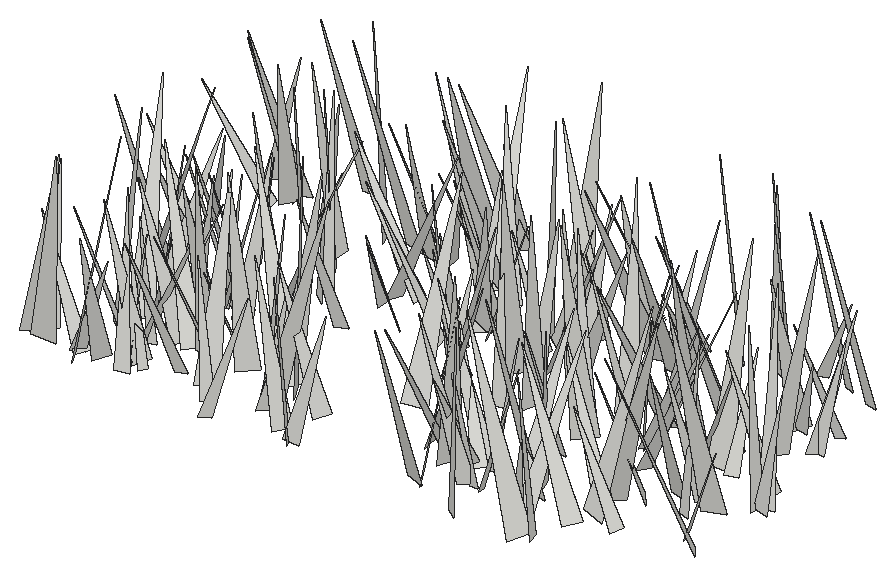
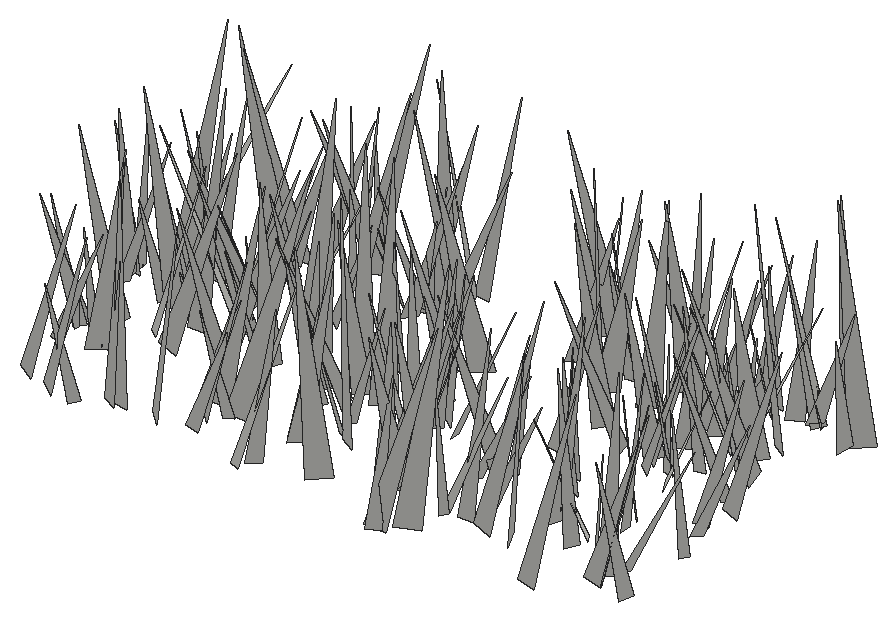
# SketchUp Ruby script. Lengths in inches.
U = 1.inch
M = Sketchup.active_model
def pt(a) = Geom::Point3d.new(a.map { |v| v * U })
def face(e, loops, mat)
  f = e.add_face(loops[0].map { |a| pt(a) })
  loops[1..].each { |l| e.add_face(l.map { |a| pt(a) }).erase! }
  f.material = f.back_material = mat if mat
  f
end
# faces: each face lists its corners as indices into pts; further lists are holes
def faces(e, pts, list, mat = nil) = list.each { |f| face(e, (f[0].is_a?(Array) ? f : [f]).map { |l| l.map { |i| pts[i] } }, mat) }
# xy, xz, yz: faces in a plane at the given z, y or x. An outline is a flat list of corners, or four numbers for a rectangle; further outlines are holes
def ring(l) = l.size == 4 ? [[l[0], l[1]], [l[2], l[1]], [l[2], l[3]], [l[0], l[3]]] : l.each_slice(2).to_a
def flat(e, list, mat, &to3) = list.each { |f| face(e, (f[0].is_a?(Array) ? f : [f]).map { |l| ring(l).map { |u, v| to3.(u, v) } }, mat) }
def xy(e, z, list, mat = nil) = flat(e, list, mat) { |x, y| [x, y, z] }
def xz(e, y, list, mat = nil) = flat(e, list, mat) { |x, z| [x, y, z] }
def yz(e, x, list, mat = nil) = flat(e, list, mat) { |y, z| [x, y, z] }
def lines(e, pts, list) = list.each { |a, b| e.add_line(pt(pts[a]), pt(pts[b])) }
# prism: a flat outline (further loops are holes) pulled along v
def prism(e, loops, v, mat = nil)
  f = face(e, loops, mat); d = Geom::Vector3d.new(v.map { |x| x * U })
  f.pushpull(f.normal.samedirection?(d) ? d.length : -d.length)
end
def box(e, o, s, mat = nil) = prism(e, [[o, [o[0] + s[0], o[1], o[2]], [o[0] + s[0], o[1] + s[1], o[2]], [o[0], o[1] + s[1], o[2]]]], [0, 0, s[2]], mat)
def at(x, y, z, deg = 0) = Geom::Transformation.translation(pt([x, y, z])) * Geom::Transformation.rotation(ORIGIN, Z_AXIS, deg.degrees)
def axes(o, x, y, z) = Geom::Transformation.new([*x, 0, *y, 0, *z, 0, *pt(o).to_a, 1])
def part(name) = M.definitions.add(name)
# library, detail: a bought-in or finely detailed component or shape, given as its bounding box
def library(name, o, s) = part(name).tap { |d| box(d.entities, o, s) }
def detail(e, o, s) = box(e.add_group.entities, o, s)
def put(e, d, t, mat = nil) = e.add_instance(d, t).tap { |i| i.material = mat if mat }
def group(e, t, mat = nil) = e.add_group.tap { |g| g.transformation = t; g.material = mat if mat }.entities
root = M.entities
c1 = part("fur_instance\#9")
p = [[0.8125,0,1.79],[0.67,-0.02,1.48],[0,-0.11,0],[0,0.11,0]]
faces(c1.entities,p,[[0,1,2,3]])
put(root,c1,axes([529.7,255.59,-21.66],[-1.86711,-6.21996,0.83765],[-6.21183,1.95621,0.67975],[0.89595,0.60083,6.45848]))
put(root,c1,axes([505.19,255.6,-21.66],[4.3108,-3.69492,0.61953],[-3.55093,-4.33068,-1.12044],[-1.19463,-0.46051,5.56597]))
put(root,c1,axes([539.13,253.99,-21.66],[-7.00283,2.97011,1.6591],[3.21934,7.01289,1.03394],[1.10002,-1.61605,7.53606]))
put(root,c1,axes([500.92,255.19,-21.66],[1.84601,-7.44066,1.73932],[-7.59322,-1.58595,1.27441],[0.85535,1.97933,7.55956]))
put(root,c1,axes([499.92,255.59,-21.66],[4.60789,-6.31495,1.14074],[-6.41656,-4.51508,0.92427],[0.08686,1.46561,7.76253]))
put(root,c1,axes([534.02,253.74,-21.66],[3.38997,4.6985,2.258],[4.82742,-3.84601,0.75539],[-1.96736,-1.34115,5.74432]))
put(root,c1,axes([514.75,253.74,-21.66],[3.82826,-1.89723,1.31218],[-2.241,-3.66166,1.2438],[-0.54703,1.72325,4.08754]))
put(root,c1,axes([503.53,255.34,-21.66],[3.31192,-3.28223,0.0309],[-3.2384,-3.26025,0.79144],[0.53549,0.5836,4.59516]))
put(root,c1,axes([520.81,254.58,-21.66],[1.98838,-4.24744,1.75797],[-4.57109,-1.62434,1.24561],[0.4862,2.09896,4.52138]))
put(root,c1,axes([520.7,254.41,-21.66],[-4.62696,-2.40171,1.71965],[-2.7299,4.69747,-0.78458],[1.12828,1.51649,5.15378]))
put(root,c1,axes([539.83,254.45,-21.66],[-4.89428,-1.48699,1.50253],[-1.73277,4.99254,-0.70337],[1.21087,1.13406,5.0666]))
put(root,c1,axes([537.2,256.21,-21.66],[0.94706,-3.59902,0.23008],[-3.53322,-0.8783,0.80484],[0.72266,0.42244,3.63347]))
put(root,c1,axes([519.43,255.46,-21.66],[-4.54367,3.48057,1.82928],[3.81076,4.58683,0.73803],[0.96889,-1.71821,5.67579]))
put(root,c1,axes([503.85,255.37,-21.66],[-3.48001,3.233,0.8636],[3.33945,3.27515,1.19585],[-0.21495,-1.45934,4.59703]))
put(root,c1,axes([529.92,255.99,-21.66],[6.22111,3.48137,1.76986],[3.77865,-6.20685,-1.07301],[-0.98698,-1.81924,7.04775]))
put(root,c1,axes([510.18,257.15,-21.66],[-0.32554,-5.06602,0.7464],[-4.99056,0.14633,-1.18345],[-1.14716,0.80105,4.9366]))
put(root,c1,axes([513.71,255.28,-21.66],[-0.78367,4.54033,1.31363],[4.69244,0.5877,0.76808],[-0.56674,-1.41222,4.54299]))
put(root,c1,axes([503.8,254.6,-21.66],[6.26441,4.08516,1.86388],[4.05019,-6.52197,0.68206],[-1.9387,-0.42509,7.44756]))
put(root,c1,axes([507.48,256.67,-21.66],[-4.95355,2.49117,1.9463],[2.93301,4.97148,1.10159],[1.17959,-1.90003,5.43416]))
put(root,c1,axes([507.28,254.95,-21.66],[-0.20928,5.81187,1.2771],[5.90875,0.05179,0.73257],[-0.70395,-1.2931,5.76932]))
put(root,c1,axes([532.45,257.21,-21.66],[0.82361,-5.861,1.93807],[-5.93962,-1.28507,-1.3621],[-1.68178,1.66825,5.75972]))
put(root,c1,axes([506.9,256.625,-21.66],[-4.69197,-2.31538,0.05263],[-2.28134,4.60011,-1.00642],[-0.39908,0.92541,5.13447]))
put(root,c1,axes([508.08,255.99,-21.66],[-3.93894,0.78438,0.2139],[0.7314,3.88076,-0.76228],[0.35506,0.70765,3.94328]))
put(root,c1,axes([531.32,259.23,-21.66],[3.03189,-3.59681,0.02756],[-3.43565,-2.90654,-1.37057],[-1.06494,-0.8632,4.50011]))
put(root,c1,axes([510.91,259.46,-21.66],[-3.83453,-4.44323,0.31037],[-4.29048,3.7947,1.3169],[1.19597,-0.63261,5.71941]))
put(root,c1,axes([506.93,255.87,-21.66],[2.12896,3.50938,0.78952],[3.35263,-2.26833,1.04217],[-1.30344,-0.10245,3.97015]))
put(root,c1,axes([533.06,257.12,-21.66],[0.75971,3.71481,1.88794],[3.89435,-1.31575,1.02184],[-1.48263,-1.55251,3.65142]))
put(root,c1,axes([517.31,256.875,-21.66],[7.2049,-3.47591,1.96261],[-3.83046,-7.15988,1.38131],[-1.1231,2.12096,7.87937]))
put(root,c1,axes([529.9,258.76,-21.66],[6.97183,-3.45055,1.53762],[-3.37643,-7.13932,-0.71191],[-1.69419,0.0288,7.74635]))
put(root,c1,axes([529.5,259.22,-21.66],[-1.20375,-5.21342,0.24756],[-5.17288,1.15789,-0.76855],[-0.69453,0.4118,5.2951]))
put(root,c1,axes([540.64,257.33,-21.66],[-4.45803,3.98436,0.74293],[4.03358,4.25341,1.39275],[-0.39655,-1.52789,5.81458]))
put(root,c1,axes([520.36,258.25,-21.66],[-4.35819,2.96505,1.59627],[3.3258,4.19926,1.28011],[0.52792,-1.97688,5.11338]))
put(root,c1,axes([512.49,256.76,-21.66],[-3.77046,5.93467,2.17976],[6.06315,4.1134,-0.71146],[1.79161,-1.43096,6.99504]))
put(root,c1,axes([536.93,258.7,-21.66],[-2.90211,-6.23156,1.67253],[-6.44447,2.71044,-1.08359],[-0.31368,1.96803,6.78825]))
put(root,c1,axes([543.29,258.36,-21.66],[-3.79672,1.89832,0.59417],[1.98792,3.66583,0.99077],[0.06937,-1.15319,4.1276]))
put(root,c1,axes([537.78,255.93,-21.66],[0.187,6.43803,0.46404],[6.40843,-0.12967,-0.78342],[0.77175,-0.48321,6.39292]))
put(root,c1,axes([516.23,257.9,-21.66],[0.00091,-3.67707,1.93886],[-4.08733,0.35251,0.67045],[0.75747,1.90654,3.61543]))
put(root,c1,axes([500.5,256.58,-21.66],[-4.9436,1.78617,0.77223],[1.56135,4.89918,-1.33648],[1.16143,1.01666,5.08364]))
put(root,c1,axes([548.65,259.28,-21.66],[-5.4011,-4.4458,0.12135],[-4.40164,5.31613,-1.14717],[-0.63674,0.96192,6.9008]))
put(root,c1,axes([533.65,257.16,-21.66],[3.84083,1.33111,0.88578],[1.09907,-3.87194,1.0529],[-1.16125,0.73803,3.92622]))
put(root,c1,axes([510.02,259.74,-21.66],[-0.4517,-7.27096,2.0225],[-7.50286,0.65147,0.6664],[0.81515,1.96726,7.25444]))
put(root,c1,axes([516.55,257.27,-21.66],[3.29752,4.92899,1.52703],[4.76096,-3.60504,1.35547],[-1.98997,-0.45731,5.77332]))
put(root,c1,axes([503.68,259.08,-21.66],[4.80804,6.17674,2.98381],[6.78482,-4.81897,-0.95722],[-1.01068,-2.96612,7.76873]))
put(root,c1,axes([536.38,259.86,-21.66],[5.52429,1.58059,2.16664],[1.98524,-5.74559,-0.8703],[-1.80317,-1.48335,5.67966]))
put(root,c1,axes([527.5,260.02,-21.66],[7.30646,0.41261,0.41525],[0.46932,-7.23653,-1.06747],[-0.34987,-1.09065,7.23983]))
put(root,c1,axes([536.5,257.24,-21.66],[-1.23708,6.4323,0.84499],[6.38548,1.35924,-0.99849],[1.14637,-0.62994,6.47363]))
put(root,c1,axes([513.18,259.92,-21.66],[3.99451,-5.40043,2.70776],[-5.64329,-4.49426,-0.63847],[-2.15638,1.75774,6.68679]))
put(root,c1,axes([506.53,258.8125,-21.66],[0.17252,3.92598,1.26935],[3.97591,-0.49782,0.99933],[-1.10305,-1.18034,3.80058]))
put(root,c1,axes([507.77,260.11,-21.66],[-5.02237,2.51021,1.68016],[2.86774,4.98644,1.12241],[0.94877,-1.78398,5.50142]))
put(root,c1,axes([539.04,259.47,-21.66],[-4.27231,-1.94809,0.06255],[-1.87913,4.07681,-1.37844],[-0.51754,1.27912,4.48861]))
put(root,c1,axes([505.97,258.65,-21.66],[4.9565,-0.0282,0.53243],[-0.1703,-4.80111,1.33099],[-0.50525,1.34155,4.77453]))
put(root,c1,axes([547,260.55,-21.66],[4.10425,1.09153,0.3293],[1.14011,-3.92312,-1.20584],[0.00571,-1.24998,4.07214]))
put(root,c1,axes([541.01,258.87,-21.66],[1.96643,7.28816,1.86053],[7.47956,-1.69089,-1.28167],[0.79683,-2.11408,7.43918]))
put(root,c1,axes([511.16,261.6,-21.66],[-2.38013,-2.88459,0.25848],[-2.75196,2.35686,0.96161],[0.90246,-0.42079,3.61403]))
put(root,c1,axes([517.23,259.52,-21.66],[6.18055,4.14964,3.19418],[4.26505,-6.85588,0.65402],[-3.03836,-1.18276,7.41558]))
put(root,c1,axes([541.47,259.5625,-21.66],[-3.45745,4.3845,0.64107],[4.38114,3.2607,1.32749],[-0.66366,-1.31634,5.42361]))
put(root,c1,axes([540.75,261.18,-21.66],[6.79044,-4.4332,0.71146],[-4.48312,-6.76549,0.63187],[-0.24718,0.91888,8.0848]))
put(root,c1,axes([531.81,259.29,-21.66],[-2.66965,3.73747,0.14274],[3.69986,2.61324,0.77338],[-0.54785,-0.56423,4.52743]))
put(root,c1,axes([531.67,260.2,-21.66],[-5.56985,2.38046,0.65327],[2.45077,5.52546,0.76123],[0.29505,-0.95874,6.00918]))
put(root,c1,axes([508.24,262.47,-21.66],[4.15376,-5.21591,0.7578],[-5.12927,-4.22232,-0.94677],[-1.21268,-0.00681,6.60024]))
put(root,c1,axes([542.1875,262.52,-21.66],[-3.97091,-3.72473,0.66515],[-3.58252,4.01146,1.07602],[1.21718,-0.34456,5.33703]))
put(root,c1,axes([508.82,259.92,-21.66],[-4.49285,4.90641,0.97236],[5.00159,4.41981,0.80831],[0.04935,-1.26349,6.60342]))
put(root,c1,axes([516.4375,260.02,-21.66],[-5.45873,5.352,1.02249],[5.44819,5.38274,0.9113],[0.08123,-1.36725,7.5902]))
put(root,c1,axes([532.74,259.44,-21.66],[1.96135,3.70682,0.36248],[3.45553,-1.96392,1.38604],[-1.38968,0.34826,3.95807]))
put(root,c1,axes([503.99,262.3125,-21.66],[3.91302,0.34843,0.25725],[0.41449,-3.69091,-1.30566],[-0.12562,-1.32482,3.70519]))
put(root,c1,axes([505.79,261.09,-21.66],[4.04604,3.23344,0.3968],[3.2461,-3.94826,-0.92578],[0.27467,-0.96906,5.09593]))
put(root,c1,axes([546.5,263.85,-21.66],[1.61042,-7.88282,1.5376],[-7.97737,-1.75156,-0.62458],[-0.92985,1.37466,8.02136]))
put(root,c1,axes([543.62,264.0625,-21.66],[-0.77388,-5.77446,0.46112],[-5.72229,0.83441,0.84559],[0.90132,0.33953,5.76439]))
put(root,c1,axes([503.95,260.98,-21.66],[-5.29033,5.65073,1.03717],[5.57546,5.38985,-0.92613],[1.38587,-0.11308,7.68509]))
put(root,c1,axes([513.87,263.45,-21.66],[5.12868,-4.19399,1.94705],[-4.5125,-5.17419,0.74098],[-1.00889,1.82269,6.58361]))
put(root,c1,axes([545.2,264.38,-21.66],[0.47741,-4.86513,1.33169],[-4.92648,-0.73691,-0.92606],[-1.08291,1.20759,4.79999]))
put(root,c1,axes([534.81,263.68,-21.66],[0.7235,3.49331,2.20248],[3.65755,-1.58024,1.30491],[-1.91742,-1.69623,3.32022]))
put(root,c1,axes([505.73,264.24,-21.66],[-0.80392,-5.00028,1.94874],[-5.12712,1.2977,1.21465],[1.58527,1.66129,4.91668]))
put(root,c1,axes([503.87,262.83,-21.66],[4.42151,2.80893,1.55928],[2.73673,-4.68252,0.67492],[-1.68278,-0.23477,5.19464]))
put(root,c1,axes([545.27,262.42,-21.66],[2.35955,4.93164,1.36493],[4.86886,-2.62618,1.07189],[-1.57426,-0.73054,5.36093]))
put(root,c1,axes([502.5,262.875,-21.66],[7.43833,2.19546,1.23858],[2.06036,-7.51855,0.95355],[-1.45225,0.57818,7.69672]))
put(root,c1,axes([509.09,264.95,-21.66],[-2.70694,-4.99144,1.16007],[-5.08628,2.45713,-1.29614],[-0.62448,1.62351,5.52829]))
put(root,c1,axes([507.4,264.74,-21.66],[5.27684,1.71083,0.85913],[1.8324,-5.24307,-0.81398],[-0.55438,-1.04563,5.4872]))
put(root,c1,axes([523.9,262.75,-21.66],[-2.77927,7.20298,1.80131],[7.21654,3.07297,-1.15349],[1.74623,-1.2353,7.63392]))
put(root,c1,axes([507.19,265.65,-21.66],[-1.65671,-3.63214,1.3485],[-3.6613,1.94738,0.7471],[1.26719,0.87797,3.92161]))
put(root,c1,axes([534.58,266.15,-21.66],[4.88048,-6.02987,2.56967],[-6.14977,-5.32095,-0.80587],[-2.26779,1.4525,7.7155]))
put(root,c1,axes([508.95,264.625,-21.66],[3.9195,-3.82723,2.46639],[-4.43668,-3.94163,0.93419],[-1.02305,2.43088,5.39791]))
put(root,c1,axes([548.6875,265.67,-21.66],[0.22976,-4.49295,1.68417],[-4.67204,0.17468,1.10336],[1.09322,1.69077,4.36142]))
put(root,c1,axes([524.9375,264.5,-21.66],[6.05583,0.88682,1.38397],[0.67013,-6.15634,1.01257],[-1.50092,0.82941,6.03608]))
put(root,c1,axes([508.51,266.19,-21.66],[-2.89225,-3.68575,0.79235],[-3.76683,2.78458,-0.79678],[-0.15371,1.11313,4.61682]))
put(root,c1,axes([511.09,265.11,-21.66],[6.06997,0.80019,0.53139],[0.73411,-6.05703,0.73529],[-0.61948,0.66277,6.07817]))
put(root,c1,axes([539.79,265.375,-21.66],[5.54197,-0.978,0.47716],[-1.05474,-5.437,1.10644],[-0.26776,1.17482,5.51777]))
put(root,c1,axes([514.28,267.65,-21.66],[0.3349,-5.08877,0.86463],[-5.08924,-0.4702,-0.79617],[-0.86188,0.79915,5.03725]))
put(root,c1,axes([529.61,267.36,-21.66],[6.66168,-2.88093,2.18206],[-2.80757,-7.00677,-0.67958],[-2.27567,0.211,7.22605]))
put(root,c1,axes([500.96,267.26,-21.66],[-1.48365,-5.76059,1.44193],[-5.8771,1.21156,-1.20691],[-0.85046,1.67706,5.82486]))
put(root,c1,axes([548.28,265.86,-21.66],[-5.81537,-0.03657,1.70774],[-0.23888,6.01751,-0.6846],[1.69135,0.72416,5.77505]))
put(root,c1,axes([507.2,265.26,-21.66],[1.88548,3.67223,0.79609],[3.49899,-2.04056,1.12569],[-1.36969,-0.15771,3.97154]))
put(root,c1,axes([523.89,267.72,-21.66],[0.22156,-4.52657,1.23949],[-4.53883,-0.5223,-1.09609],[-1.19379,1.1457,4.39744]))
put(root,c1,axes([548.08,267.77,-21.66],[-5.1344,0.67452,1.09766],[0.89094,5.11676,1.02317],[0.93062,-1.17714,5.07643]))
put(root,c1,axes([506.37,266.86,-21.66],[-4.07706,-2.14403,0.24298],[-2.12817,3.90987,-1.20919],[-0.35608,1.18084,4.44491]))
put(root,c1,axes([501.99,266.1875,-21.66],[0.82135,5.31818,1.14764],[5.3338,-0.55827,-1.23031],[1.07271,-1.29616,5.2387]))
put(root,c1,axes([501.57,269.32,-21.66],[1.96703,-4.29578,0.10046],[-4.18734,-1.94112,-1.01553],[-0.96439,-0.33368,4.61429]))
put(root,c1,axes([527.99,265.95,-21.66],[0.38602,5.6901,1.15392],[5.67114,-0.61727,1.14668],[-1.24374,-1.04858,5.58671]))
put(root,c1,axes([523.28,266.94,-21.66],[-1.54021,3.23682,1.39983],[3.28512,1.87235,-0.71486],[1.28237,-0.90889,3.51258]))
put(root,c1,axes([540.67,269.62,-21.66],[-0.69616,-7.71222,1.47846],[-7.81205,0.83092,0.65597],[0.79755,1.40715,7.71575]))
put(root,c1,axes([541.72,268.75,-21.66],[4.55769,0.07164,0.01251],[0.0727,-4.46545,-0.91231],[0.00209,-0.91239,4.46602]))
put(root,c1,axes([548.7,266.15,-21.66],[0.5538,7.06628,1.29605],[7.05626,-0.7792,1.23321],[-1.34954,-1.17443,6.97985]))
put(root,c1,axes([538.15,267.66,-21.66],[4.95013,-1.23925,0.4471],[-1.29852,-4.88303,0.8422],[-0.22245,0.9272,5.03291]))
put(root,c1,axes([537.6,270.55,-21.66],[0.04578,-6.29285,0.19538],[-6.21134,-0.07706,-1.02644],[-1.02831,0.18529,6.20874]))
put(root,c1,axes([526.07,269.75,-21.66],[5.79688,-5.3049,1.7816],[-5.31494,-6.02201,-0.63769],[-1.75142,0.71643,7.83193]))
put(root,c1,axes([538.76,267.92,-21.66],[6.16739,3.42449,0.19717],[3.4017,-6.05394,-1.25736],[0.441,-1.19388,6.94138]))
put(root,c1,axes([522.88,268.21,-21.66],[0.28684,-3.45624,1.82339],[-3.70035,-0.82791,-0.9872],[-1.25608,1.64973,3.32465]))
put(root,c1,axes([521.8,269.97,-21.66],[4.64418,-2.47093,1.08294],[-2.19439,-4.71399,-1.3452],[-1.56935,-0.72073,5.0857]))
put(root,c1,axes([538.14,267.4,-21.66],[2.54415,2.86578,1.34064],[2.68524,-2.86561,1.02977],[-1.67317,-0.2414,3.6912]))
put(root,c1,axes([517.02,269.83,-21.66],[-2.4025,-2.92839,0.44923],[-2.80853,2.4353,0.85486],[0.94311,-0.20767,3.69008]))
put(root,c1,axes([536.98,268.03,-21.66],[-5.93557,-1.05009,0.32847],[-1.08922,5.86272,-0.94003],[0.15548,0.98355,5.95399]))
put(root,c1,axes([511.06,269.55,-21.66],[-1.26744,-3.38882,1.28492],[-3.35573,1.6115,0.94004],[1.36901,0.81271,3.49382]))
put(root,c1,axes([520.22,270.07,-21.66],[-4.86082,-0.82699,0.28427],[-0.77768,4.82218,0.73078],[0.39992,-0.67448,4.87621]))
put(root,c1,axes([543.32,268.33,-21.66],[-0.77106,7.66776,2.67234],[8.04873,1.0768,-0.76736],[1.07416,-2.56446,7.66813]))
put(root,c1,axes([521.7,268.93,-21.66],[-3.13424,-4.33981,2.11732],[-4.81159,3.01955,-0.93345],[0.40688,2.2779,5.27125]))
put(root,c1,axes([544.48,268.05,-21.66],[-1.99149,3.68652,0.84504],[3.6319,2.13053,-0.73532],[1.05538,-0.37542,4.12502]))
put(root,c1,axes([542.64,271.51,-21.66],[-3.72414,-4.2026,0.59605],[-4.10843,3.76818,0.89886],[1.06672,-0.15915,5.54285]))
put(root,c1,axes([527.93,269.5,-21.66],[3.39124,-4.48702,2.29298],[-4.9912,-3.37077,0.78574],[-0.69206,2.32297,5.56924]))
put(root,c1,axes([535.83,267.92,-21.66],[3.94824,4.29759,0.4959],[4.2386,-3.97723,0.72087],[-0.86569,0.12707,5.79122]))
put(root,c1,axes([531.21,269.27,-21.66],[-0.70822,-5.57958,3.0516],[-6.3293,0.31925,-0.88519],[-0.61961,3.1164,5.55425]))
put(root,c1,axes([532.92,268.48,-21.66],[-5.60196,1.71083,0.59088],[1.59688,5.57635,-1.00614],[0.85208,0.79713,5.77032]))
put(root,c1,axes([514.48,271.57,-21.66],[3.47774,-1.50181,0.39234],[-1.2719,-3.30895,-1.39185],[-0.88975,-1.13996,3.5232]))
put(root,c1,axes([500.89,270.55,-21.66],[-4.33776,1.46199,0.55548],[1.55819,4.18055,1.16497],[0.13425,-1.28363,4.42678]))
put(root,c1,axes([530.15,270.73,-21.66],[5.34451,-3.5502,0.35957],[-3.55754,-5.25077,1.03462],[0.27778,1.05952,6.33224]))
put(root,c1,axes([505.1,271.22,-21.66],[2.93725,2.51058,1.33666],[2.80043,-2.8887,-0.72813],[-0.49727,-1.43859,3.79478]))
put(root,c1,axes([540.76,272.54,-21.66],[-1.61608,-6.86234,1.14057],[-6.89566,1.42577,-1.19223],[-0.91789,1.37106,6.94853]))
put(root,c1,axes([521.15,272.77,-21.66],[2.32461,-5.72045,0.33614],[-5.68592,-2.25756,0.90225],[0.71192,0.64824,6.10846]))
put(root,c1,axes([534.47,270.4375,-21.66],[-6.2785,3.87073,1.88034],[3.7817,6.55006,-0.85632],[2.05354,-0.22787,7.32591]))
put(root,c1,axes([504.8,272.67,-21.66],[-4.71927,-1.33587,1.95814],[-1.09743,5.09822,0.83318],[2.10107,-0.33763,4.83341]))
put(root,c1,axes([499.81,273.16,-21.66],[4.41728,-0.60705,0.29796],[-0.51929,-4.30631,-1.07505],[-0.43316,-1.02804,4.32726]))
put(root,c1,axes([521.92,272.57,-21.66],[4.65437,1.55789,0.49043],[1.62302,-4.57734,-0.86283],[-0.1826,-0.97553,4.83174]))
put(root,c1,axes([526.16,272.83,-21.66],[-4.20728,0.83557,0.99678],[1.00115,4.23485,0.67581],[0.83033,-0.87227,4.23588]))
put(root,c1,axes([534.18,271.43,-21.66],[4.3038,1.80689,1.01933],[1.67441,-4.41138,0.75005],[-1.22483,0.31842,4.60705]))
put(root,c1,axes([510.49,270.9,-21.66],[0.64289,6.12986,1.03372],[6.0316,-0.86662,1.38779],[-1.50455,-0.85491,6.00521]))
put(root,c1,axes([545.08,271.88,-21.66],[6.61649,-1.70465,2.3436],[-2.13195,-6.81989,1.0584],[-1.96294,1.66119,6.75008]))
put(root,c1,axes([515.89,273.36,-21.66],[-4.18794,0.93567,0.33129],[0.9893,4.05153,1.06324],[0.08071,-1.11073,4.15738]))
put(root,c1,axes([514.51,272.54,-21.66],[6.16079,-1.33707,0.34037],[-1.37023,-6.11166,0.79308],[-0.16154,0.84778,6.25413]))
put(root,c1,axes([527.73,271.25,-21.66],[6.18202,1.83786,0.77531],[1.68935,-6.16651,1.14736],[-1.06062,0.8903,6.34654]))
put(root,c1,axes([521.85,273.81,-21.66],[-1.08629,-5.09453,1.21583],[-5.17343,0.84989,-1.06105],[-0.81738,1.39139,5.09985]))
put(root,c1,axes([533.82,275.89,-21.66],[-0.13701,-6.93499,0.01519],[-6.899,0.13785,0.70555],[0.70571,0.00117,6.90036]))
put(root,c1,axes([509.59,272.91,-21.66],[4.32475,3.25099,2.86901],[3.37923,-5.06616,0.64681],[-2.71679,-1.12634,5.37159]))
put(root,c1,axes([532.06,276.6,-21.66],[1.01288,-8.11783,0.06805],[-8.08119,-1.01477,-0.77093],[-0.77341,-0.02823,8.14437]))
put(root,c1,axes([529.11,272.39,-21.66],[4.10356,-2.98524,2.70877],[-3.77942,-4.1935,1.10399],[-1.40181,2.56732,4.95298]))
put(root,c1,axes([544.13,275.28,-21.66],[4.71186,-4.25626,1.34995],[-4.06485,-4.9009,-1.26409],[-1.848,-0.07223,6.22249]))
put(root,c1,axes([546.75,273.59,-21.66],[-0.57371,3.97778,1.97621],[4.19128,1.14438,-1.08668],[1.47014,-1.71025,3.86924]))
put(root,c1,axes([508.65,274.45,-21.66],[-6.63003,0.58928,2.6026],[0.94805,7.03587,0.82207],[2.49439,-1.10786,6.6052]))
put(root,c1,axes([521.1875,272.5,-21.66],[-4.05743,3.11883,1.27429],[2.94276,4.25195,-1.03673],[1.64046,0.08657,5.0115]))
put(root,c1,axes([544.29,275.11,-21.66],[0.84418,-3.62493,0.18375],[-3.45271,-0.74384,1.18829],[1.11924,0.43944,3.52714]))
put(root,c1,axes([535.8,272.97,-21.66],[6.16496,0.12051,1.82007],[-0.27856,-6.27765,1.3592],[-1.80266,1.38221,6.01447]))
put(root,c1,axes([524.73,274.97,-21.66],[4.42565,6.01002,3.52258],[6.87552,-4.43985,-1.06317],[-1.12079,-3.50468,7.38759]))
put(root,c1,axes([525.68,274.25,-21.66],[2.6257,3.60497,0.95618],[3.72031,-2.44904,-0.98281],[0.26337,-1.34567,4.35019]))
put(root,c1,axes([546.72,273.36,-21.66],[4.55494,-1.38322,1.77977],[-1.90749,-4.50337,1.38185],[-1.20098,1.9065,4.55536]))
put(root,c1,axes([527.64,276.375,-21.66],[2.72704,-3.27265,0.76108],[-3.17295,-2.83078,-0.80329],[-1.10537,0.05182,4.1835]))
put(root,c1,axes([546.74,275.91,-21.66],[-0.5806,-4.0301,0.94816],[-3.96701,0.26756,-1.29192],[-1.18471,1.07913,3.86131]))
put(root,c1,axes([506.03,276.37,-21.66],[5.48101,-1.25937,0.85366],[-1.15676,-5.52263,-0.72019],[-0.98826,-0.52035,5.57753]))
put(root,c1,axes([505.86,274.9375,-21.66],[3.45283,2.51437,0.03768],[2.48973,-3.40925,-0.65094],[0.3531,-0.54815,4.22141]))
put(root,c1,axes([501.48,276.82,-21.66],[-4.90231,-0.23018,0.15933],[-0.18525,4.76264,1.18065],[0.20988,-1.17272,4.76358]))
put(root,c1,axes([512.93,275.78,-21.66],[-4.21656,2.08304,0.19454],[2.06998,4.09043,1.06765],[-0.30342,-1.04195,4.58024]))
put(root,c1,axes([518.06,277.62,-21.66],[-3.59271,-3.52154,0.36411],[-3.38524,3.56898,1.11534],[1.03633,-0.55007,4.90559]))
put(root,c1,axes([513.2,277.79,-21.66],[-0.67207,-6.04885,0.74296],[-6.03248,0.76649,0.78356],[0.86591,0.6451,6.03542]))
put(root,c1,axes([519.13,277.32,-21.66],[-0.74587,-6.40704,1.23448],[-6.45249,0.53969,-1.09751],[-0.96927,1.33753,6.35625]))
put(root,c1,axes([534.17,277.69,-21.66],[1.81992,-3.21241,0.00061],[-3.09433,-1.75321,-0.99152],[-0.86298,-0.48823,3.55649]))
put(root,c1,axes([502.11,277.83,-21.66],[4.76035,-4.27512,0.72339],[-4.20428,-4.81383,-0.78223],[-1.06017,-0.10597,6.35025]))
put(root,c1,axes([519.03,275.78,-21.66],[-7.32876,-0.97242,0.83606],[-1.07916,7.29688,-0.97277],[0.69283,1.07947,7.32872]))
put(root,c1,axes([511.65,278.15,-21.66],[-2.25691,-7.5793,1.44794],[-7.71352,2.17504,-0.63772],[-0.20948,1.56823,7.88243]))
put(root,c1,axes([515.05,277.23,-21.66],[-3.55918,-3.90599,0.48478],[-3.91702,3.45103,-0.95229],[-0.38568,0.99656,5.19785]))
put(root,c1,axes([527.17,276.62,-21.66],[-5.93712,3.87569,1.72238],[4.1151,5.9813,0.72589],[1.02637,-1.56207,7.0529]))
put(root,c1,axes([514.61,278.17,-21.66],[4.05285,-0.43746,0.41546],[-0.3233,-3.95717,-1.01285],[-0.50937,-0.96903,3.94856]))
put(root,c1,axes([501.86,278.57,-21.66],[-5.14482,-3.13912,1.24988],[-3.04737,5.29445,0.7535],[1.4594,-0.01101,5.97959]))
put(root,c1,axes([503.72,276.93,-21.66],[-3.72029,-1.54775,1.40082],[-1.82397,3.80239,-0.64288],[1.01535,1.15959,3.97778]))
put(root,c1,axes([520.62,276.35,-21.66],[-2.14866,5.91991,1.32548],[6.06222,2.04254,0.70466],[-0.22751,-1.48381,6.25824]))
put(root,c1,axes([533.73,277.67,-21.66],[-3.99562,-4.42007,1.47298],[-4.65768,3.83659,-1.12173],[0.11293,1.84803,5.85182]))
put(root,c1,axes([532.43,276.95,-21.66],[-0.05946,3.80591,1.08242],[3.88392,0.26301,-0.71143],[0.75616,-1.05166,3.7393]))
put(root,c1,axes([515.28,280.91,-21.66],[4.78768,-6.87101,0.53821],[-6.76798,-4.81092,-1.21319],[-1.30189,-0.25808,8.28619]))
put(root,c1,axes([502.28,279.05,-21.66],[-0.64276,-5.9949,1.38637],[-6.03632,0.34404,-1.31091],[-1.1932,1.48889,5.88502]))
put(root,c1,axes([533.38,279.33,-21.66],[-0.33962,-4.53633,0.58104],[-4.49375,0.22275,-0.88758],[-0.84975,0.63509,4.46159]))
put(root,c1,axes([509.49,278.01,-21.66],[-6.31517,-2.67121,2.41272],[-3.08957,6.52254,-0.86542],[1.84694,1.77736,6.80204]))
put(root,c1,axes([528.45,281.37,-21.66],[-3.25593,-5.45811,0.05054],[-5.36708,3.21208,1.12765],[0.99394,-0.53501,6.25464]))
put(root,c1,axes([539.3,280.02,-21.66],[-3.95013,-6.45103,2.53754],[-6.55598,4.42551,1.04517],[2.25256,1.56763,7.49179]))
put(root,c1,axes([538.61,279.94,-21.66],[-1.6159,-6.90986,2.38073],[-7.13771,2.01606,1.00679],[1.57067,2.05292,7.0245]))
put(root,c1,axes([527.76,280.32,-21.66],[3.7662,-3.06911,1.25827],[-2.92554,-3.97067,-0.92842],[-1.56328,0.03677,4.76883]))
put(root,c1,axes([523.4,279.39,-21.66],[-3.8242,6.03816,3.67075],[6.53219,4.61268,-0.78232],[2.69524,-2.61192,7.10435]))
put(root,c1,axes([499.39,279.3,-21.66],[4.23339,-1.74729,1.15695],[-1.93705,-4.25778,0.65751],[-0.79963,1.0637,4.53236]))
put(root,c1,axes([518.63,277.12,-21.66],[-3.78371,6.02543,0.57396],[5.96039,3.82698,-0.88298],[1.05307,-0.01122,7.05993]))
put(root,c1,axes([545.73,280.2,-21.66],[-2.90009,-5.61636,1.60668],[-5.82709,2.65472,-1.23809],[-0.41218,1.98605,6.19848]))
put(root,c1,axes([535.98,279.7,-21.66],[3.85266,4.81198,3.39076],[5.17881,-4.69725,0.78179],[-2.79863,-2.06788,6.11449]))
put(root,c1,axes([516.89,282.08,-21.66],[1.34944,-6.66989,1.0863],[-6.57389,-1.5523,-1.36482],[-1.56569,0.76902,6.66676]))
put(root,c1,axes([505.28,281.82,-21.66],[-1.29627,-6.42722,1.30707],[-6.54569,1.18361,-0.67151],[-0.41416,1.4099,6.52216]))
put(root,c1,axes([516.8,282.33,-21.66],[3.0521,-3.8403,0.46149],[-3.78154,-3.08617,-0.67208],[-0.8129,-0.06212,4.85917]))
put(root,c1,axes([541.03,281.27,-21.66],[2.68666,-2.71893,0.01615],[-2.65256,-2.616,0.85524],[0.59729,0.61233,3.72549]))
put(root,c1,axes([543.38,281.01,-21.66],[-3.32572,-4.76152,1.64129],[-5.0351,3.09772,-1.21581],[-0.11678,2.03921,5.67929]))
